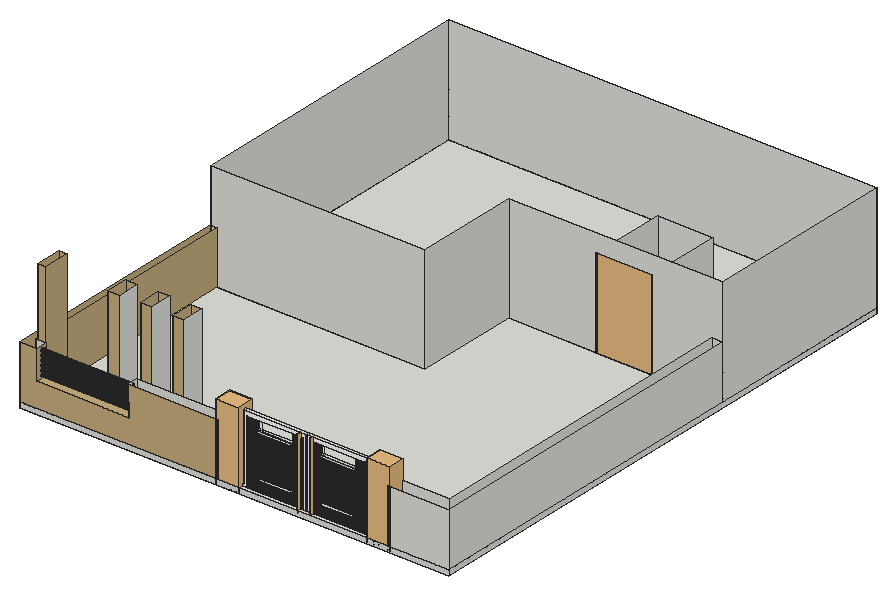
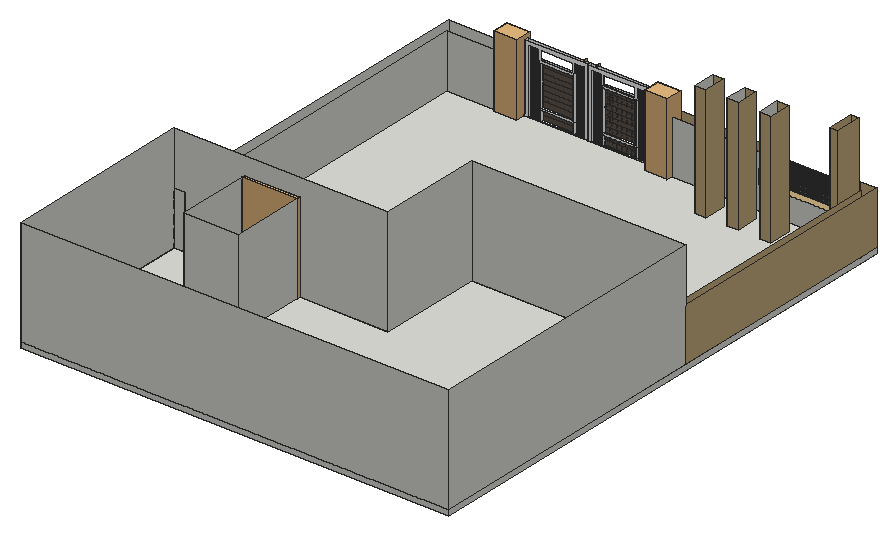
# SketchUp Ruby script. Lengths in inches.
U = 1.inch
M = Sketchup.active_model
def pt(a) = Geom::Point3d.new(a.map { |v| v * U })
def face(e, loops, mat)
  f = e.add_face(loops[0].map { |a| pt(a) })
  loops[1..].each { |l| e.add_face(l.map { |a| pt(a) }).erase! }
  f.material = f.back_material = mat if mat
  f
end
# faces: each face lists its corners as indices into pts; further lists are holes
def faces(e, pts, list, mat = nil) = list.each { |f| face(e, (f[0].is_a?(Array) ? f : [f]).map { |l| l.map { |i| pts[i] } }, mat) }
# xy, xz, yz: faces in a plane at the given z, y or x. An outline is a flat list of corners, or four numbers for a rectangle; further outlines are holes
def ring(l) = l.size == 4 ? [[l[0], l[1]], [l[2], l[1]], [l[2], l[3]], [l[0], l[3]]] : l.each_slice(2).to_a
def flat(e, list, mat, &to3) = list.each { |f| face(e, (f[0].is_a?(Array) ? f : [f]).map { |l| ring(l).map { |u, v| to3.(u, v) } }, mat) }
def xy(e, z, list, mat = nil) = flat(e, list, mat) { |x, y| [x, y, z] }
def xz(e, y, list, mat = nil) = flat(e, list, mat) { |x, z| [x, y, z] }
def yz(e, x, list, mat = nil) = flat(e, list, mat) { |y, z| [x, y, z] }
def lines(e, pts, list) = list.each { |a, b| e.add_line(pt(pts[a]), pt(pts[b])) }
# prism: a flat outline (further loops are holes) pulled along v
def prism(e, loops, v, mat = nil)
  f = face(e, loops, mat); d = Geom::Vector3d.new(v.map { |x| x * U })
  f.pushpull(f.normal.samedirection?(d) ? d.length : -d.length)
end
def box(e, o, s, mat = nil) = prism(e, [[o, [o[0] + s[0], o[1], o[2]], [o[0] + s[0], o[1] + s[1], o[2]], [o[0], o[1] + s[1], o[2]]]], [0, 0, s[2]], mat)
def at(x, y, z, deg = 0) = Geom::Transformation.translation(pt([x, y, z])) * Geom::Transformation.rotation(ORIGIN, Z_AXIS, deg.degrees)
def axes(o, x, y, z) = Geom::Transformation.new([*x, 0, *y, 0, *z, 0, *pt(o).to_a, 1])
def part(name) = M.definitions.add(name)
# library, detail: a bought-in or finely detailed component or shape, given as its bounding box
def library(name, o, s) = part(name).tap { |d| box(d.entities, o, s) }
def detail(e, o, s) = box(e.add_group.entities, o, s)
def put(e, d, t, mat = nil) = e.add_instance(d, t).tap { |i| i.material = mat if mat }
def group(e, t, mat = nil) = e.add_group.tap { |g| g.transformation = t; g.material = mat if mat }.entities
root = M.entities
M.materials.add("[0134_DimGray]").color = [105, 105, 105]
M.materials.add("[Color_000]").color = [255, 255, 255]
M.materials.add("[Color_C20]").color = [102, 91, 81]
M.materials.add("[Roofing Slate Tan]").color = [200, 175, 128]
c1 = library("Gate pillar",[0,0,0],[97.06,71.13,326.45])
c2 = library("Gate pull handle",[-0.01,0,0],[1.26,2.875,48])
c3 = part("Horizontal gate slat")
xy(c3.entities,0,[[0.39,114.16,6.3,114.17]])
xy(c3.entities,0,[[0.39,0,6.3,114.16]],"[Color_C20]")
xy(c3.entities,0.39,[[0.39,0,0.79,114.17],[0.98,0,2.07,114.17],[2.36,0,3.2,114.17],[3.59,0,4.37,114.17],[4.56,0,5.71,114.17],
  [5.91,0,6.3,114.17]],"[Color_C20]")
xy(c3.entities,0.79,[[0.39,0,0.79,114.17],[0.98,0,2.07,114.17],[2.36,0,3.2,114.17],[3.59,0,4.37,114.17],[4.56,0,5.71,114.17],
  [5.91,0,6.3,114.17]],"[Color_C20]")
xy(c3.entities,0.99,[[1.13,0,1.21,114.16],[1.87,0,1.94,114.16],[2.61,0,2.68,114.16],[3.35,0,3.42,114.16],[4.08,0,4.16,114.16],
  [4.82,0,4.9,114.16],[5.5625,0,5.63,114.16],[6.3,0,6.37,114.16]],"[Color_C20]")
xy(c3.entities,1.18,[[0.39,114.16,3.35,114.17],[3.35,114.16,6.3,114.17]])
xy(c3.entities,1.18,[[0.39,0,1.13,114.16],[1.21,0,1.87,114.16],[1.94,0,2.61,114.16],[2.68,0,3.35,114.16],[3.42,0,4.08,114.16],
  [4.16,0,4.82,114.16],[4.9,0,5.5625,114.16],[5.63,0,6.3,114.16]],"[Color_C20]")
xz(c3.entities,0,[[[0.39,0,6.3,0,6.3,0.39,5.91,0.39,5.91,0.79,6.3,0.79,6.3,1.18,5.63,1.18,5.63,0.99,5.5625,0.99,5.5625,1.18,4.9,1.18,4.9,0.99,4.82,0.99,4.82,1.18,4.16,1.18,4.16,0.99,4.08,0.99,4.08,1.18,3.42,1.18,3.42,0.99,3.35,0.99,3.35,1.18,2.68,1.18,2.68,0.99,2.61,0.99,2.61,1.18,1.94,1.18,1.94,0.99,1.87,0.99,1.87,1.18,1.21,1.18,1.21,0.99,1.13,0.99,1.13,1.18,0.39,1.18,0.39,0.79,0.79,0.79,0.79,0.39,0.39,0.39],[4.56,0.39,5.71,0.79],[0.98,0.39,2.07,0.79],[2.36,0.39,3.2,0.79],[3.59,0.39,4.37,0.79]],[6.3,0.99,6.37,1.18]],"[Color_C20]")
xz(c3.entities,114.16,[[1.13,0.99,1.21,1.18],[1.87,0.99,1.94,1.18],[2.61,0.99,2.68,1.18],[3.35,0.99,3.42,1.18],[4.08,0.99,4.16,1.18],
  [4.82,0.99,4.9,1.18],[5.5625,0.99,5.63,1.18]],"[Color_C20]")
xz(c3.entities,114.17,[[[0.39,0,0.39,0.39,0.79,0.39,0.79,0.79,0.39,0.79,0.39,1.18,6.3,1.18,6.3,0.79,5.91,0.79,5.91,0.39,6.3,0.39,6.3,0],[4.56,0.39,5.71,0.79],[0.98,0.39,2.07,0.79],[2.36,0.39,3.2,0.79],[3.59,0.39,4.37,0.79]]],"[Color_C20]")
yz(c3.entities,0.39,[[114.16,0,114.17,0.39],[114.16,0.79,114.17,1.18]])
yz(c3.entities,0.39,[[0,0,114.16,0.39],[0,0.79,114.16,1.18]],"[Color_C20]")
yz(c3.entities,0.79,[[0,0.39,114.17,0.79]],"[Color_C20]")
yz(c3.entities,0.98,[[0,0.39,114.17,0.79]],"[Color_C20]")
yz(c3.entities,1.13,[[0,0.99,114.16,1.18]],"[Color_C20]")
yz(c3.entities,1.21,[[0,0.99,114.16,1.18]],"[Color_C20]")
yz(c3.entities,1.87,[[0,0.99,114.16,1.18]],"[Color_C20]")
yz(c3.entities,1.94,[[0,0.99,114.16,1.18]],"[Color_C20]")
yz(c3.entities,2.07,[[0,0.39,114.17,0.79]],"[Color_C20]")
yz(c3.entities,2.36,[[0,0.39,114.17,0.79]],"[Color_C20]")
yz(c3.entities,2.61,[[0,0.99,114.16,1.18]],"[Color_C20]")
yz(c3.entities,2.68,[[0,0.99,114.16,1.18]],"[Color_C20]")
yz(c3.entities,3.2,[[0,0.39,114.17,0.79]],"[Color_C20]")
yz(c3.entities,3.35,[[0,0.99,114.16,1.18]],"[Color_C20]")
yz(c3.entities,3.42,[[0,0.99,114.16,1.18]],"[Color_C20]")
yz(c3.entities,3.59,[[0,0.39,114.17,0.79]],"[Color_C20]")
yz(c3.entities,4.08,[[0,0.99,114.16,1.18]],"[Color_C20]")
yz(c3.entities,4.16,[[0,0.99,114.16,1.18]],"[Color_C20]")
yz(c3.entities,4.37,[[0,0.39,114.17,0.79]],"[Color_C20]")
yz(c3.entities,4.56,[[0,0.39,114.17,0.79]],"[Color_C20]")
yz(c3.entities,4.82,[[0,0.99,114.16,1.18]],"[Color_C20]")
yz(c3.entities,4.9,[[0,0.99,114.16,1.18]],"[Color_C20]")
yz(c3.entities,5.5625,[[0,0.99,114.16,1.18]],"[Color_C20]")
yz(c3.entities,5.63,[[0,0.99,114.16,1.18]],"[Color_C20]")
yz(c3.entities,5.71,[[0,0.39,114.17,0.79]],"[Color_C20]")
yz(c3.entities,5.91,[[0,0.39,114.17,0.79]],"[Color_C20]")
yz(c3.entities,6.3,[[114.16,0,114.17,0.39],[114.16,0.79,114.17,1.18]])
yz(c3.entities,6.3,[[0,0,114.16,0.39],[0,0.79,114.16,0.99],[0,0.99,114.16,1.18]],"[Color_C20]")
yz(c3.entities,6.37,[[0,0.99,114.16,1.18]],"[Color_C20]")
p = [[0,0,0],[0.39,0,0]]
lines(c3.entities,p,[[0,1]])
c4 = part("Vertical gate panel")
put(c4.entities,c3,axes([0,1.18,0],[3.67755,0,0],[0,0,2.40086],[0,-1,0]))
put(c4.entities,c3,axes([21.72,1.18,0],[3.67755,0,0],[0,0,2.40086],[0,-1,0]))
c5 = library("PINTU 6 YA",[0,-0.6875,0],[35.83,8.07,80.71])
xy(root,-6,[[0,15.9375,480,615.9375]])
xy(root,-5.25,[[387.83,22.11,387.69,22.13,387.57,22.18,387.47,22.25,387.38,22.35,387.33,22.46,387.32,22.59,387.33,22.71,387.38,22.82,387.47,22.92,387.57,23,387.69,23.05,387.83,23.0625,387.96,23.05,388.08,23,388.18,22.92,388.27,22.82,388.32,22.71,388.33,22.59,388.32,22.46,388.27,22.35,388.18,22.25,388.08,22.18,387.96,22.13],[246.02,22.23,245.89,22.24,245.77,22.29,245.66,22.375,245.58,22.48,245.53,22.6,245.51,22.73,245.53,22.87,245.58,22.99,245.66,23.09,245.77,23.17,245.89,23.23,246.02,23.24,246.15,23.23,246.27,23.17,246.38,23.09,246.46,22.99,246.51,22.87,246.53,22.73,246.51,22.6,246.46,22.48,246.38,22.375,246.27,22.29,246.15,22.24]])
xy(root,-3.69,[[[243.87,20.54,316.77,24.42],[246.02,22.23,246.15,22.24,246.27,22.29,246.38,22.375,246.46,22.48,246.51,22.6,246.53,22.73,246.51,22.87,246.46,22.99,246.38,23.09,246.27,23.17,246.15,23.23,246.02,23.24,245.89,23.23,245.77,23.17,245.66,23.09,245.58,22.99,245.53,22.87,245.51,22.73,245.53,22.6,245.58,22.48,245.66,22.375,245.77,22.29,245.89,22.24]],[[317.07,20.54,388.6,24.16],[387.83,22.11,387.96,22.13,388.08,22.18,388.18,22.25,388.27,22.35,388.32,22.46,388.33,22.59,388.32,22.71,388.27,22.82,388.18,22.92,388.08,23,387.96,23.05,387.83,23.0625,387.69,23.05,387.57,23,387.47,22.92,387.38,22.82,387.33,22.71,387.32,22.59,387.33,22.46,387.38,22.35,387.47,22.25,387.57,22.18,387.69,22.13]]],"[Color_000]")
xy(root,0,[[0,15.9375,0,283.1875,6.6875,283.1875,6.6875,28.66,221.75,28.66,221.75,15.9375],[[221.75,15.9375,221.75,28.66,6.6875,28.66,6.6875,283.1875,240,283.1875,240,400.0625,339.53,400.0625,339.53,485.1875,401.28,485.1875,401.28,400.0625,468.66,400.0625,468.66,32.24,411.91,32.24,411.91,15.9375],[149.98,42.13,162.73,67.13],[113.7,42.13,126.45,67.13],[77.42,42.13,90.17,67.13],[7.64,30.94,16.14,60.82]],[411.91,15.9375,411.91,32.24,468.66,32.24,468.66,400.0625,480,400.0625,480,15.9375],[0,283.1875,0,615.9375,480,615.9375,480,400.0625,401.28,400.0625,401.28,485.1875,339.53,485.1875,339.53,400.0625,240,400.0625,240,283.1875]])
xy(root,0.34,[[261.95,20.54,263.68,21.1875],[263.68,20.54,299.69,21.1875],[299.69,20.54,301.41,21.1875],[332.43,20.54,334.15,21.14],[334.15,20.54,370.17,21.14],
  [370.17,20.54,371.89,21.14]])
xy(root,0.34,[[250.625,20.54,256.29,24.42],[256.29,20.54,261.95,24.42],[301.41,20.54,312.74,21.1875],[321.1,20.54,332.43,21.14],[371.89,20.54,377.56,24.16],
  [377.56,20.54,383.22,24.16],[321.1,21.14,332.43,24.16],[334.15,21.14,370.17,24.16],[263.68,21.1875,299.69,24.42],[301.41,21.1875,312.74,24.42]],"[Color_000]")
xy(root,1.87,[[243.87,20.54,246.59,24.42],[387.25,20.54,388.6,24.16]],"[Color_000]")
xy(root,11.67,[[263.68,20.54,299.69,24.42],[334.15,20.54,370.17,24.16]],"[Color_000]")
xy(root,13.39,[[263.68,20.54,299.69,24.42],[334.15,20.54,370.17,24.16]],"[Color_000]")
xy(root,27.125,[[18.32,15.9375,122.09,28.66]],"[Roofing Slate Tan]")
xy(root,59.22,[[263.68,20.54,299.69,24.42],[334.15,20.54,370.17,24.16]],"[Color_000]")
xz(root,15.9375,[[0,-6,480,0],[411.91,0,480,60]])
xz(root,15.9375,[[0,0,221.75,0,221.75,60,120.04,60,122.09,27.125,18.32,27.125,18.32,60,0,60]],"[Roofing Slate Tan]")
xz(root,20.54,[[[243.87,-3.69,316.77,-3.69,316.77,76.3,246.59,76.3,246.59,1.87,243.87,1.87],[250.625,0.34,312.74,72.27]],[[317.07,-3.69,388.6,-3.69,388.6,1.87,387.25,1.87,387.25,76.3,317.07,76.3],[321.1,0.34,383.22,72.27]],[261.95,0.34,263.68,11.67],[299.69,0.34,301.41,11.67],[332.43,0.34,334.15,11.67],
  [370.17,0.34,371.89,11.67],[261.95,11.67,301.41,11.67,301.41,60.9375,261.95,60.9375,261.95,59.22,299.69,59.22,299.69,13.39,263.68,13.39,263.68,59.22,261.95,59.22],[332.43,11.67,371.89,11.67,371.89,59.22,370.17,59.22,370.17,13.39,334.15,13.39,334.15,59.22,371.89,59.22,371.89,60.9375,332.43,60.9375]],"[Color_000]")
xz(root,24.16,[[[317.07,-3.69,317.07,76.3,387.25,76.3,387.25,1.87,388.6,1.87,388.6,-3.69],[334.15,13.39,370.17,59.22],[371.89,0.34,383.22,72.27],[321.1,0.34,332.43,72.27],[334.15,60.9375,370.17,72.27],[334.15,0.34,370.17,11.67]]],"[Color_000]")
xz(root,24.42,[[[243.87,-3.69,243.87,1.87,246.59,1.87,246.59,76.3,316.77,76.3,316.77,-3.69],[263.68,13.39,299.69,59.22],[250.625,0.34,261.95,72.27],[301.41,0.34,312.74,72.27],[263.68,60.9375,299.69,72.27],[263.68,0.34,299.69,11.67]]],"[Color_000]")
xz(root,28.66,[[6.6875,0,6.6875,60,18.32,60,18.32,27.125,122.09,27.125,120.04,60,221.75,60,221.75,0]])
xz(root,30.94,[[7.64,0,16.14,134.54]],"[Roofing Slate Tan]")
xz(root,32.24,[[411.91,0,468.66,60]])
xz(root,42.13,[[77.42,0,90.17,126.8125],[113.7,0,126.45,128],[149.98,0,162.73,128]],"[Roofing Slate Tan]")
xz(root,60.82,[[7.64,0,16.14,134.54]],"[Roofing Slate Tan]")
xz(root,67.13,[[77.42,0,90.17,126.8125],[113.7,0,126.45,128],[149.98,0,162.73,128]],"[Roofing Slate Tan]")
xz(root,283.1875,[[0,0,6.6875,60],[6.6875,0,240,0,240,120,0,120,0,60,6.6875,60]])
xz(root,400.0625,[[240,0,339.53,0,339.53,99.91,401.28,99.91,401.28,0,468.66,0,468.66,60,480,60,480,120,240,120],[468.66,0,480,60]])
xz(root,485.1875,[[339.53,0,401.28,99.91]])
xz(root,615.9375,[[0,-6,480,0],[0,0,480,120]])
yz(root,0,[[15.9375,-6,615.9375,0],[283.1875,0,615.9375,120]])
yz(root,0,[[15.9375,0,283.1875,60]],"[Roofing Slate Tan]")
yz(root,6.6875,[[28.66,0,283.1875,60]],"[Roofing Slate Tan]")
yz(root,7.64,[[30.94,0,60.82,134.54]],"[Roofing Slate Tan]")
yz(root,16.14,[[30.94,0,60.82,134.54]],"[Roofing Slate Tan]")
yz(root,18.32,[[[15.9375,27.125,28.66,60],[23.05,34.27,22.61,34.29,22.1875,34.43,21.82,34.66,21.52,34.99,21.32,35.38,21.23,35.8125,21.25,36.25,21.39,36.67,21.625,37.04,21.95,37.34,22.34,37.54,22.77,37.63,23.21,37.61,23.63,37.48,24,37.24,24.3,36.91,24.5,36.52,24.59,36.09,24.57,35.65,24.44,35.23,24.2,34.86,23.87,34.5625,23.48,34.36],[23.05,39.28,22.61,39.3,22.1875,39.4375,21.82,39.68,21.52,40,21.32,40.4,21.23,40.83,21.25,41.27,21.39,41.6875,21.625,42.06,21.95,42.35,22.34,42.55,22.77,42.64,23.21,42.62,23.63,42.49,24,42.25,24.3,41.92,24.5,41.53,24.59,41.1,24.57,40.66,24.44,40.24,24.2,39.87,23.87,39.57,23.48,39.375],[23.05,49.31,22.61,49.33,22.1875,49.46,21.82,49.7,21.52,50.03,21.32,50.42,21.23,50.85,21.25,51.29,21.39,51.71,21.625,52.08,21.95,52.375,22.34,52.58,22.77,52.67,23.21,52.65,23.63,52.51,24,52.27,24.3,51.95,24.5,51.55,24.59,51.125,24.57,50.68,24.44,50.26,24.2,49.89,23.87,49.6,23.48,49.4],[23.05,54.32,22.61,54.34,22.1875,54.48,21.82,54.71,21.52,55.04,21.32,55.43,21.23,55.86,21.25,56.3,21.39,56.72,21.625,57.09,21.95,57.39,22.34,57.59,22.77,57.68,23.21,57.66,23.63,57.53,24,57.29,24.3,56.96,24.5,56.57,24.59,56.14,24.57,55.7,24.44,55.28,24.2,54.91,23.87,54.61,23.48,54.41],[23.05,29.26,22.61,29.28,22.1875,29.41,21.82,29.65,21.52,29.98,21.32,30.37,21.23,30.8,21.25,31.24,21.39,31.66,21.625,32.03,21.95,32.33,22.34,32.53,22.77,32.62,23.21,32.6,23.63,32.46,24,32.22,24.3,31.9,24.5,31.5,24.59,31.07,24.57,30.63,24.44,30.21,24.2,29.84,23.87,29.55,23.48,29.35],[23.05,44.29,22.61,44.32,22.1875,44.45,21.82,44.69,21.52,45.02,21.32,45.41,21.23,45.84,21.25,46.28,21.39,46.7,21.625,47.07,21.95,47.36,22.34,47.56,22.77,47.66,23.21,47.64,23.63,47.5,24,47.26,24.3,46.93,24.5,46.54,24.59,46.11,24.57,45.67,24.44,45.25,24.2,44.88,23.87,44.59,23.48,44.39]]],"[Roofing Slate Tan]")
yz(root,77.42,[[42.13,0,67.13,126.8125]],"[Roofing Slate Tan]")
yz(root,90.17,[[42.13,0,67.13,126.8125]])
yz(root,113.7,[[42.13,0,67.13,128]],"[Roofing Slate Tan]")
yz(root,120.52,[[23.05,54.32,23.48,54.41,23.87,54.61,24.2,54.91,24.44,55.28,24.57,55.7,24.59,56.14,24.5,56.57,24.3,56.96,24,57.29,23.63,57.53,23.21,57.66,22.77,57.68,22.34,57.59,21.95,57.39,21.625,57.09,21.39,56.72,21.25,56.3,21.23,55.86,21.32,55.43,21.52,55.04,21.82,54.71,22.1875,54.48,22.61,54.34]])
yz(root,121.0625,[[23.05,39.28,23.48,39.375,23.87,39.57,24.2,39.87,24.44,40.24,24.57,40.66,24.59,41.1,24.5,41.53,24.3,41.92,24,42.25,23.63,42.49,23.21,42.62,22.77,42.64,22.34,42.55,21.95,42.35,21.625,42.06,21.39,41.6875,21.25,41.27,21.23,40.83,21.32,40.4,21.52,40,21.82,39.68,22.1875,39.4375,22.61,39.3]])
yz(root,121.5,[[23.05,29.26,23.48,29.35,23.87,29.55,24.2,29.84,24.44,30.21,24.57,30.63,24.59,31.07,24.5,31.5,24.3,31.9,24,32.22,23.63,32.46,23.21,32.6,22.77,32.62,22.34,32.53,21.95,32.33,21.625,32.03,21.39,31.66,21.25,31.24,21.23,30.8,21.32,30.37,21.52,29.98,21.82,29.65,22.1875,29.41,22.61,29.28],[23.05,34.27,23.48,34.36,23.87,34.5625,24.2,34.86,24.44,35.23,24.57,35.65,24.59,36.09,24.5,36.52,24.3,36.91,24,37.24,23.63,37.48,23.21,37.61,22.77,37.63,22.34,37.54,21.95,37.34,21.625,37.04,21.39,36.67,21.25,36.25,21.23,35.8125,21.32,35.38,21.52,34.99,21.82,34.66,22.1875,34.43,22.61,34.29]])
yz(root,122.51,[[23.05,49.31,23.48,49.4,23.87,49.6,24.2,49.89,24.44,50.26,24.57,50.68,24.59,51.125,24.5,51.55,24.3,51.95,24,52.27,23.63,52.51,23.21,52.65,22.77,52.67,22.34,52.58,21.95,52.375,21.625,52.08,21.39,51.71,21.25,51.29,21.23,50.85,21.32,50.42,21.52,50.03,21.82,49.7,22.1875,49.46,22.61,49.33]])
yz(root,123.45,[[23.05,44.29,23.48,44.39,23.87,44.59,24.2,44.88,24.44,45.25,24.57,45.67,24.59,46.11,24.5,46.54,24.3,46.93,24,47.26,23.63,47.5,23.21,47.64,22.77,47.66,22.34,47.56,21.95,47.36,21.625,47.07,21.39,46.7,21.25,46.28,21.23,45.84,21.32,45.41,21.52,45.02,21.82,44.69,22.1875,44.45,22.61,44.32]])
yz(root,126.45,[[42.13,0,67.13,128]])
yz(root,149.98,[[42.13,0,67.13,128]],"[Roofing Slate Tan]")
yz(root,162.73,[[42.13,0,67.13,128]])
yz(root,221.75,[[15.9375,0,28.66,60]])
yz(root,240,[[283.1875,0,400.0625,120]])
yz(root,243.87,[[20.54,-3.69,24.42,1.87]],"[Color_000]")
yz(root,246.59,[[[20.54,1.87,24.42,76.3],[21.91,61.26,23.37,64],[21.91,65.08,23.37,67.71],[21.91,64.12,23.37,64.95]]],"[Color_000]")
yz(root,250.625,[[20.54,0.34,24.42,72.27]],"[Color_000]")
yz(root,261.95,[[20.54,0.34,24.42,11.67],[20.54,11.67,24.42,59.22],[20.54,59.22,24.42,60.9375]],"[Color_000]")
yz(root,263.68,[[20.54,0.34,24.42,11.67],[20.54,13.39,24.42,59.22]],"[Color_000]")
yz(root,299.69,[[20.54,0.34,24.42,11.67],[20.54,13.39,24.42,59.22]],"[Color_000]")
yz(root,301.41,[[20.54,0.34,24.42,11.67],[20.54,11.67,24.42,60.9375]],"[Color_000]")
yz(root,312.74,[[20.54,0.34,24.42,72.27]],"[Color_000]")
yz(root,316.77,[[20.54,-3.69,24.42,76.3]],"[Color_000]")
yz(root,317.07,[[20.54,-3.69,24.16,76.3]],"[Color_000]")
yz(root,321.1,[[20.54,0.34,24.16,72.27]],"[Color_000]")
yz(root,332.43,[[20.54,0.34,24.16,11.67],[20.54,11.67,24.16,60.9375]],"[Color_000]")
yz(root,334.15,[[20.54,0.34,24.16,11.67],[20.54,13.39,24.16,59.22]],"[Color_000]")
yz(root,339.53,[[400.0625,0,485.1875,99.91]])
yz(root,370.17,[[20.54,0.34,24.16,11.67],[20.54,13.39,24.16,59.22]],"[Color_000]")
yz(root,371.89,[[20.54,0.34,24.16,11.67],[20.54,11.67,24.16,59.22],[20.54,59.22,24.16,60.9375]],"[Color_000]")
yz(root,383.22,[[20.54,0.34,24.16,72.27]],"[Color_000]")
yz(root,387.25,[[[20.54,1.87,24.16,76.3],[21.82,61.26,21.82,64,23.18,64,23.18,64.12,21.82,64.12,21.82,64.95,23.18,64.95,23.18,61.26],[21.82,65.08,23.18,67.71]]],"[Color_000]")
yz(root,388.6,[[20.54,-3.69,24.16,1.87]],"[Color_000]")
yz(root,401.28,[[400.0625,0,485.1875,99.91]])
yz(root,411.91,[[15.9375,0,32.24,60]])
yz(root,468.66,[[32.24,0,400.0625,60]])
yz(root,480,[[15.9375,-6,615.9375,0],[15.9375,0,400.0625,60],[400.0625,0,615.9375,120]])
p = [[387.69,22.13,-3.69],[387.57,22.18,-3.69],[387.57,22.18,-5.25],[387.69,22.13,-5.25],[387.83,22.11,-3.69],[387.83,22.11,-5.25],
  [387.96,22.13,-3.69],[387.96,22.13,-5.25],[388.08,22.18,-3.69],[388.08,22.18,-5.25],[245.89,22.24,-3.69],[245.77,22.29,-3.69],
  [245.77,22.29,-5.25],[245.89,22.24,-5.25],[246.02,22.23,-3.69],[246.02,22.23,-5.25],[246.15,22.24,-3.69],[246.15,22.24,-5.25],
  [246.27,22.29,-3.69],[246.27,22.29,-5.25],[387.47,22.25,-3.69],[387.47,22.25,-5.25],[388.18,22.25,-3.69],[388.18,22.25,-5.25],
  [245.66,22.375,-3.69],[245.66,22.375,-5.25],[246.38,22.375,-3.69],[246.38,22.375,-5.25],[387.38,22.35,-3.69],[387.38,22.35,-5.25],
  [388.27,22.35,-3.69],[388.27,22.35,-5.25],[245.58,22.48,-3.69],[245.58,22.48,-5.25],[246.46,22.48,-3.69],[246.46,22.48,-5.25],
  [387.33,22.46,-3.69],[387.33,22.46,-5.25],[388.32,22.46,-3.69],[388.32,22.46,-5.25],[245.53,22.6,-3.69],[245.53,22.6,-5.25],
  [246.51,22.6,-3.69],[246.51,22.6,-5.25],[387.32,22.59,-3.69],[387.32,22.59,-5.25],[388.33,22.59,-3.69],[388.33,22.59,-5.25],
  [245.51,22.73,-3.69],[245.51,22.73,-5.25],[246.53,22.73,-3.69],[246.53,22.73,-5.25],[387.33,22.71,-3.69],[387.33,22.71,-5.25],
  [388.32,22.71,-3.69],[388.32,22.71,-5.25],[245.53,22.87,-3.69],[245.53,22.87,-5.25],[246.51,22.87,-3.69],[246.51,22.87,-5.25],
  [387.38,22.82,-3.69],[387.38,22.82,-5.25],[388.27,22.82,-3.69],[388.27,22.82,-5.25],[387.47,22.92,-3.69],[387.47,22.92,-5.25],
  [388.18,22.92,-3.69],[388.18,22.92,-5.25],[245.58,22.99,-3.69],[245.58,22.99,-5.25],[246.46,22.99,-3.69],[246.46,22.99,-5.25],
  [387.57,23,-3.69],[387.57,23,-5.25],[388.08,23,-3.69],[388.08,23,-5.25],[245.66,23.09,-3.69],[245.66,23.09,-5.25],
  [246.38,23.09,-3.69],[246.38,23.09,-5.25],[387.69,23.05,-3.69],[387.69,23.05,-5.25],[387.83,23.0625,-3.69],[387.83,23.0625,-5.25],
  [387.96,23.05,-3.69],[387.96,23.05,-5.25],[245.77,23.17,-3.69],[245.77,23.17,-5.25],[246.27,23.17,-3.69],[246.27,23.17,-5.25],
  [245.89,23.23,-3.69],[245.89,23.23,-5.25],[246.02,23.24,-3.69],[246.02,23.24,-5.25],[246.15,23.23,-3.69],[246.15,23.23,-5.25],
  [122.09,15.9375,27.125],[120.04,15.9375,60],[120.04,28.66,60],[122.09,28.66,27.125],[18.32,22.1875,29.41],[18.32,22.61,29.28],
  [121.5,22.61,29.28],[121.5,22.1875,29.41],[18.32,23.05,29.26],[121.5,23.05,29.26],[18.32,23.48,29.35],[121.5,23.48,29.35],
  [18.32,23.87,29.55],[121.5,23.87,29.55],[18.32,21.82,29.65],[121.5,21.82,29.65],[18.32,24.2,29.84],[121.5,24.2,29.84],
  [18.32,21.52,29.98],[121.5,21.52,29.98],[18.32,24.44,30.21],[121.5,24.44,30.21],[18.32,21.32,30.37],[121.5,21.32,30.37],
  [18.32,24.57,30.63],[121.5,24.57,30.63],[18.32,21.23,30.8],[121.5,21.23,30.8],[18.32,24.59,31.07],[121.5,24.59,31.07],
  [18.32,21.25,31.24],[121.5,21.25,31.24],[18.32,24.5,31.5],[121.5,24.5,31.5],[18.32,21.39,31.66],[121.5,21.39,31.66],
  [18.32,24.3,31.9],[121.5,24.3,31.9],[18.32,21.625,32.03],[121.5,21.625,32.03],[18.32,24,32.22],[121.5,24,32.22],
  [18.32,21.95,32.33],[121.5,21.95,32.33],[18.32,23.63,32.46],[121.5,23.63,32.46],[18.32,22.34,32.53],[121.5,22.34,32.53],
  [18.32,22.77,32.62],[121.5,22.77,32.62],[18.32,23.21,32.6],[121.5,23.21,32.6],[18.32,22.1875,34.43],[18.32,22.61,34.29],
  [121.5,22.61,34.29],[121.5,22.1875,34.43],[18.32,23.05,34.27],[121.5,23.05,34.27],[18.32,23.48,34.36],[121.5,23.48,34.36],
  [18.32,21.82,34.66],[121.5,21.82,34.66],[18.32,23.87,34.5625],[121.5,23.87,34.5625],[18.32,24.2,34.86],[121.5,24.2,34.86],
  [18.32,21.52,34.99],[121.5,21.52,34.99],[18.32,24.44,35.23],[121.5,24.44,35.23],[18.32,21.32,35.38],[121.5,21.32,35.38],
  [18.32,24.57,35.65],[121.5,24.57,35.65],[18.32,21.23,35.8125],[121.5,21.23,35.8125],[18.32,24.59,36.09],[121.5,24.59,36.09],
  [18.32,21.25,36.25],[121.5,21.25,36.25],[18.32,24.5,36.52],[121.5,24.5,36.52],[18.32,21.39,36.67],[121.5,21.39,36.67],
  [18.32,24.3,36.91],[121.5,24.3,36.91],[18.32,21.625,37.04],[121.5,21.625,37.04],[18.32,24,37.24],[121.5,24,37.24],
  [18.32,21.95,37.34],[121.5,21.95,37.34],[18.32,23.63,37.48],[121.5,23.63,37.48],[18.32,22.34,37.54],[121.5,22.34,37.54],
  [18.32,22.77,37.63],[121.5,22.77,37.63],[18.32,23.21,37.61],[121.5,23.21,37.61],[18.32,22.1875,39.4375],[18.32,22.61,39.3],
  [121.0625,22.61,39.3],[121.0625,22.1875,39.4375],[18.32,23.05,39.28],[121.0625,23.05,39.28],[18.32,23.48,39.375],[121.0625,23.48,39.375],
  [18.32,21.82,39.68],[121.0625,21.82,39.68],[18.32,23.87,39.57],[121.0625,23.87,39.57],[18.32,24.2,39.87],[121.0625,24.2,39.87],
  [18.32,21.52,40],[121.0625,21.52,40],[18.32,24.44,40.24],[121.0625,24.44,40.24],[18.32,21.32,40.4],[121.0625,21.32,40.4],
  [18.32,24.57,40.66],[121.0625,24.57,40.66],[18.32,21.23,40.83],[121.0625,21.23,40.83],[18.32,24.59,41.1],[121.0625,24.59,41.1],
  [18.32,21.25,41.27],[121.0625,21.25,41.27],[18.32,24.5,41.53],[121.0625,24.5,41.53],[18.32,21.39,41.6875],[121.0625,21.39,41.6875],
  [18.32,24.3,41.92],[121.0625,24.3,41.92],[18.32,21.625,42.06],[121.0625,21.625,42.06],[18.32,24,42.25],[121.0625,24,42.25],
  [18.32,21.95,42.35],[121.0625,21.95,42.35],[18.32,23.63,42.49],[121.0625,23.63,42.49],[18.32,22.34,42.55],[121.0625,22.34,42.55],
  [18.32,23.21,42.62],[121.0625,23.21,42.62],[18.32,22.77,42.64],[121.0625,22.77,42.64],[18.32,22.1875,44.45],[18.32,22.61,44.32],
  [123.45,22.61,44.32],[123.45,22.1875,44.45],[18.32,23.05,44.29],[123.45,23.05,44.29],[18.32,23.48,44.39],[123.45,23.48,44.39],
  [18.32,23.87,44.59],[123.45,23.87,44.59],[18.32,21.82,44.69],[123.45,21.82,44.69],[18.32,24.2,44.88],[123.45,24.2,44.88],
  [18.32,21.52,45.02],[123.45,21.52,45.02],[18.32,24.44,45.25],[123.45,24.44,45.25],[18.32,21.32,45.41],[123.45,21.32,45.41],
  [18.32,24.57,45.67],[123.45,24.57,45.67],[18.32,21.23,45.84],[123.45,21.23,45.84],[18.32,24.59,46.11],[123.45,24.59,46.11],
  [18.32,21.25,46.28],[123.45,21.25,46.28],[18.32,24.5,46.54],[123.45,24.5,46.54],[18.32,21.39,46.7],[123.45,21.39,46.7],
  [18.32,24.3,46.93],[123.45,24.3,46.93],[18.32,21.625,47.07],[123.45,21.625,47.07],[18.32,24,47.26],[123.45,24,47.26],
  [18.32,21.95,47.36],[123.45,21.95,47.36],[18.32,23.63,47.5],[123.45,23.63,47.5],[18.32,22.34,47.56],[123.45,22.34,47.56],
  [18.32,23.21,47.64],[123.45,23.21,47.64],[18.32,22.77,47.66],[123.45,22.77,47.66],[18.32,22.1875,49.46],[18.32,22.61,49.33],
  [122.51,22.61,49.33],[122.51,22.1875,49.46],[18.32,23.05,49.31],[122.51,23.05,49.31],[18.32,23.48,49.4],[122.51,23.48,49.4],
  [18.32,23.87,49.6],[122.51,23.87,49.6],[18.32,21.82,49.7],[122.51,21.82,49.7],[18.32,24.2,49.89],[122.51,24.2,49.89],
  [18.32,21.52,50.03],[122.51,21.52,50.03],[18.32,24.44,50.26],[122.51,24.44,50.26],[18.32,21.32,50.42],[122.51,21.32,50.42],
  [18.32,24.57,50.68],[122.51,24.57,50.68],[18.32,21.23,50.85],[122.51,21.23,50.85],[18.32,24.59,51.125],[122.51,24.59,51.125],
  [18.32,21.25,51.29],[122.51,21.25,51.29],[18.32,24.5,51.55],[122.51,24.5,51.55],[18.32,21.39,51.71],[122.51,21.39,51.71],
  [18.32,24.3,51.95],[122.51,24.3,51.95],[18.32,21.625,52.08],[122.51,21.625,52.08],[18.32,24,52.27],[122.51,24,52.27],
  [18.32,21.95,52.375],[122.51,21.95,52.375],[18.32,23.63,52.51],[122.51,23.63,52.51],[18.32,22.34,52.58],[122.51,22.34,52.58],
  [18.32,23.21,52.65],[122.51,23.21,52.65],[18.32,22.77,52.67],[122.51,22.77,52.67],[18.32,22.1875,54.48],[18.32,22.61,54.34],
  [120.52,22.61,54.34],[120.52,22.1875,54.48],[18.32,23.05,54.32],[120.52,23.05,54.32],[18.32,23.48,54.41],[120.52,23.48,54.41],
  [18.32,23.87,54.61],[120.52,23.87,54.61],[18.32,21.82,54.71],[120.52,21.82,54.71],[18.32,24.2,54.91],[120.52,24.2,54.91],
  [18.32,21.52,55.04],[120.52,21.52,55.04],[18.32,24.44,55.28],[120.52,24.44,55.28],[18.32,21.32,55.43],[120.52,21.32,55.43],
  [18.32,24.57,55.7],[120.52,24.57,55.7],[18.32,21.23,55.86],[120.52,21.23,55.86],[18.32,24.59,56.14],[120.52,24.59,56.14],
  [18.32,21.25,56.3],[120.52,21.25,56.3],[18.32,24.5,56.57],[120.52,24.5,56.57],[18.32,21.39,56.72],[120.52,21.39,56.72],
  [18.32,24.3,56.96],[120.52,24.3,56.96],[18.32,21.625,57.09],[120.52,21.625,57.09],[18.32,24,57.29],[120.52,24,57.29],
  [18.32,21.95,57.39],[120.52,21.95,57.39],[18.32,23.63,57.53],[120.52,23.63,57.53],[18.32,22.34,57.59],[120.52,22.34,57.59],
  [18.32,23.21,57.66],[120.52,23.21,57.66],[18.32,22.77,57.68],[120.52,22.77,57.68],[203.29,53.09,-6],[437.46,53.09,-6],
  [203.29,53.09,-5.25],[437.46,53.09,-5.25],[372.6,21.14,0.34],[371.89,21.14,0.34],[370.17,21.14,61.36],[370.17,21.14,13.39],
  [261.24,21.1875,0.34],[261.95,21.1875,0.34],[263.68,21.1875,61.36],[263.68,21.1875,13.39],[316.77,20.54,-3.69],[317.07,20.54,-3.69]]
faces(root,p,[[0,1,2,3],[4,0,3,5],[6,4,5,7],[8,6,7,9],[10,11,12,13],[14,10,13,15],[16,14,15,17],[18,16,17,19],
  [1,20,21,2],[22,8,9,23],[11,24,25,12],[26,18,19,27],[20,28,29,21],[30,22,23,31],[24,32,33,25],[34,26,27,35],
  [28,36,37,29],[38,30,31,39],[32,40,41,33],[42,34,35,43],[36,44,45,37],[46,38,39,47],[40,48,49,41],[50,42,43,51],
  [44,52,53,45],[54,46,47,55],[48,56,57,49],[58,50,51,59],[52,60,61,53],[62,54,55,63],[60,64,65,61],[66,62,63,67],
  [56,68,69,57],[70,58,59,71],[64,72,73,65],[74,66,67,75],[68,76,77,69],[78,70,71,79],[72,80,81,73],[80,82,83,81],
  [82,84,85,83],[84,74,75,85],[76,86,87,77],[88,78,79,89],[86,90,91,87],[90,92,93,91],[92,94,95,93],[94,88,89,95]],"[Color_000]")
faces(root,p,[[96,97,98,99]])
faces(root,p,[[100,101,102,103],[101,104,105,102],[104,106,107,105],[106,108,109,107],[110,100,103,111],[108,112,113,109],[114,110,111,115],[112,116,117,113],
  [118,114,115,119],[116,120,121,117],[122,118,119,123],[120,124,125,121],[126,122,123,127],[124,128,129,125],[130,126,127,131],[128,132,133,129],
  [134,130,131,135],[132,136,137,133],[138,134,135,139],[136,140,141,137],[142,138,139,143],[144,142,143,145],[140,146,147,141],[146,144,145,147],
  [148,149,150,151],[149,152,153,150],[152,154,155,153],[156,148,151,157],[154,158,159,155],[158,160,161,159],[162,156,157,163],[160,164,165,161],
  [166,162,163,167],[164,168,169,165],[170,166,167,171],[168,172,173,169],[174,170,171,175],[172,176,177,173],[178,174,175,179],[176,180,181,177],
  [182,178,179,183],[180,184,185,181],[186,182,183,187],[184,188,189,185],[190,186,187,191],[192,190,191,193],[188,194,195,189],[194,192,193,195],
  [196,197,198,199],[197,200,201,198],[200,202,203,201],[204,196,199,205],[202,206,207,203],[206,208,209,207],[210,204,205,211],[208,212,213,209],
  [214,210,211,215],[212,216,217,213],[218,214,215,219],[216,220,221,217],[222,218,219,223],[220,224,225,221],[226,222,223,227],[224,228,229,225],
  [230,226,227,231],[228,232,233,229],[234,230,231,235],[232,236,237,233],[238,234,235,239],[236,240,241,237],[242,238,239,243],[240,242,243,241],
  [244,245,246,247],[245,248,249,246],[248,250,251,249],[250,252,253,251],[254,244,247,255],[252,256,257,253],[258,254,255,259],[256,260,261,257],
  [262,258,259,263],[260,264,265,261],[266,262,263,267],[264,268,269,265],[270,266,267,271],[268,272,273,269],[274,270,271,275],[272,276,277,273],
  [278,274,275,279],[276,280,281,277],[282,278,279,283],[280,284,285,281],[286,282,283,287],[284,288,289,285],[290,286,287,291],[288,290,291,289],
  [292,293,294,295],[293,296,297,294],[296,298,299,297],[298,300,301,299],[302,292,295,303],[300,304,305,301],[306,302,303,307],[304,308,309,305],
  [310,306,307,311],[308,312,313,309],[314,310,311,315],[312,316,317,313],[318,314,315,319],[316,320,321,317],[322,318,319,323],[320,324,325,321],
  [326,322,323,327],[324,328,329,325],[330,326,327,331],[328,332,333,329],[334,330,331,335],[332,336,337,333],[338,334,335,339],[336,338,339,337],
  [340,341,342,343],[341,344,345,342],[344,346,347,345],[346,348,349,347],[350,340,343,351],[348,352,353,349],[354,350,351,355],[352,356,357,353],
  [358,354,355,359],[356,360,361,357],[362,358,359,363],[360,364,365,361],[366,362,363,367],[364,368,369,365],[370,366,367,371],[368,372,373,369],
  [374,370,371,375],[372,376,377,373],[378,374,375,379],[376,380,381,377],[382,378,379,383],[380,384,385,381],[386,382,383,387],[384,386,387,385]],"[0134_DimGray]")
lines(root,p,[[388,389],[390,388],[391,389],[392,393],[394,395],[396,397],[398,399],[400,401]])
put(root,c1,axes([219.57,15.9375,-5.25],[0.2624,0,0],[0,0.2624,0],[0,0,0.2624]))
put(root,c1,axes([414.27,15.9375,-5.25],[-0.2624,0,0],[0,0.2624,0],[0,0,0.2624]))
put(root,c2,axes([324.58,17.39,-3.37],[-1.12832,0,0],[0,1.09659,0],[0,0,1.65976]))
put(root,c2,axes([309.27,17.17,-3.37],[1.12832,0,0],[0,1.1751,0],[0,0,1.65976]))
put(root,c4,axes([334.16,21.14,-0.05],[0,0,0.2676],[0,0.24487,0],[0.13139,0,0]))
put(root,c4,axes([299.6875,21.1875,-0.05],[0,0,0.2676],[0,0.2624,0],[-0.13139,0,0]))
put(root,c5,axes([338.8,400.0625,0],[1.74372,0,0],[0,0.5,0],[0,0,1.23795]))
put(root,c3,axes([383.67,21.43,0.34],[-0.96499,0,0],[0,0,0.62999],[0,-0.24487,0]))
put(root,c3,axes([377.97,21.43,0.34],[-0.96499,0,0],[0,0,0.62999],[0,-0.24487,0]))
put(root,c3,axes([327.18,21.43,0.34],[-0.96499,0,0],[0,0,0.62999],[0,-0.24487,0]))
put(root,c3,axes([332.88,21.43,0.34],[-0.96499,0,0],[0,0,0.62999],[0,-0.24487,0]))
put(root,c3,axes([250.18,21.5,0.34],[0.96499,0,0],[0,0,0.62999],[0,-0.2624,0]))
put(root,c3,axes([255.875,21.5,0.34],[0.96499,0,0],[0,0,0.62999],[0,-0.2624,0]))
put(root,c3,axes([300.97,21.5,0.34],[0.96499,0,0],[0,0,0.62999],[0,-0.2624,0]))
put(root,c3,axes([306.67,21.5,0.34],[0.96499,0,0],[0,0,0.62999],[0,-0.2624,0]))
put(root,c4,axes([334.15,21.14,13.25],[0,0,0.26237],[0,0.24487,0],[0.13139,0,0]))
put(root,c4,axes([299.7,21.1875,13.25],[0,0,0.26237],[0,0.2624,0],[-0.13139,0,0]))
put(root,c4,axes([334.15,21.14,24.65],[0,0,0.26237],[0,0.24487,0],[0.13139,0,0]))
put(root,c4,axes([299.7,21.1875,24.65],[0,0,0.26237],[0,0.2624,0],[-0.13139,0,0]))
put(root,c4,axes([334.15,21.14,36.04],[0,0,0.26237],[0,0.24487,0],[0.13139,0,0]))
put(root,c4,axes([299.69,21.1875,36.04],[0,0,0.26237],[0,0.2624,0],[-0.13139,0,0]))
put(root,c4,axes([334.15,21.14,47.44],[0,0,0.26237],[0,0.24487,0],[0.13139,0,0]))
put(root,c4,axes([299.69,21.1875,47.44],[0,0,0.26237],[0,0.2624,0],[-0.13139,0,0]))
